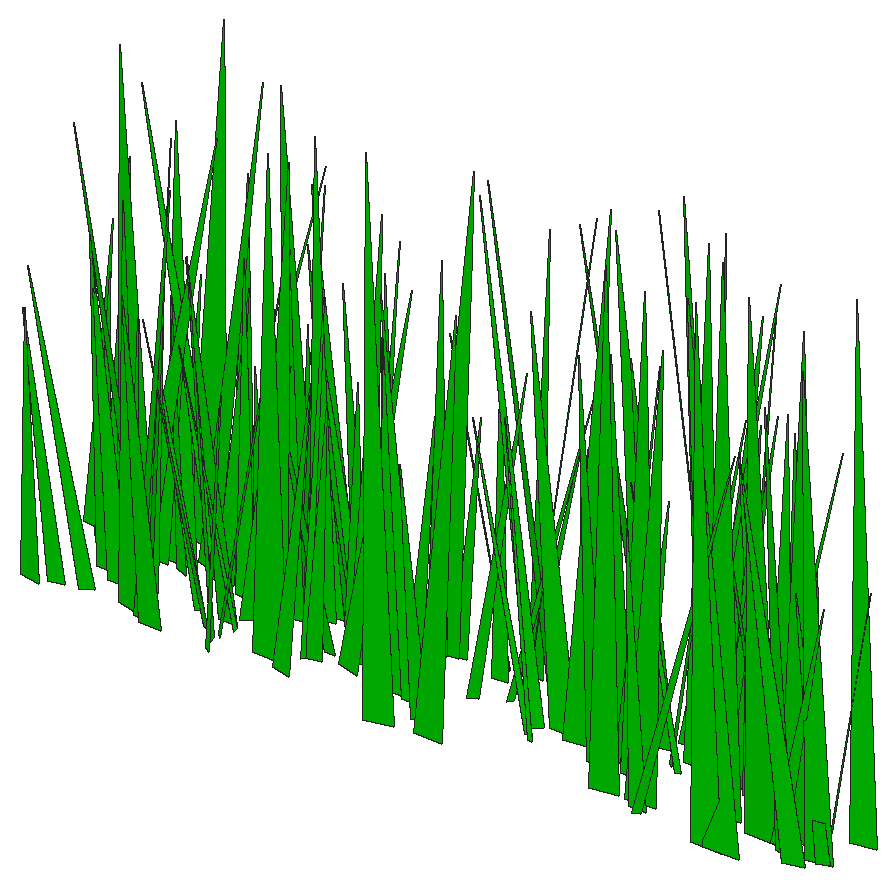
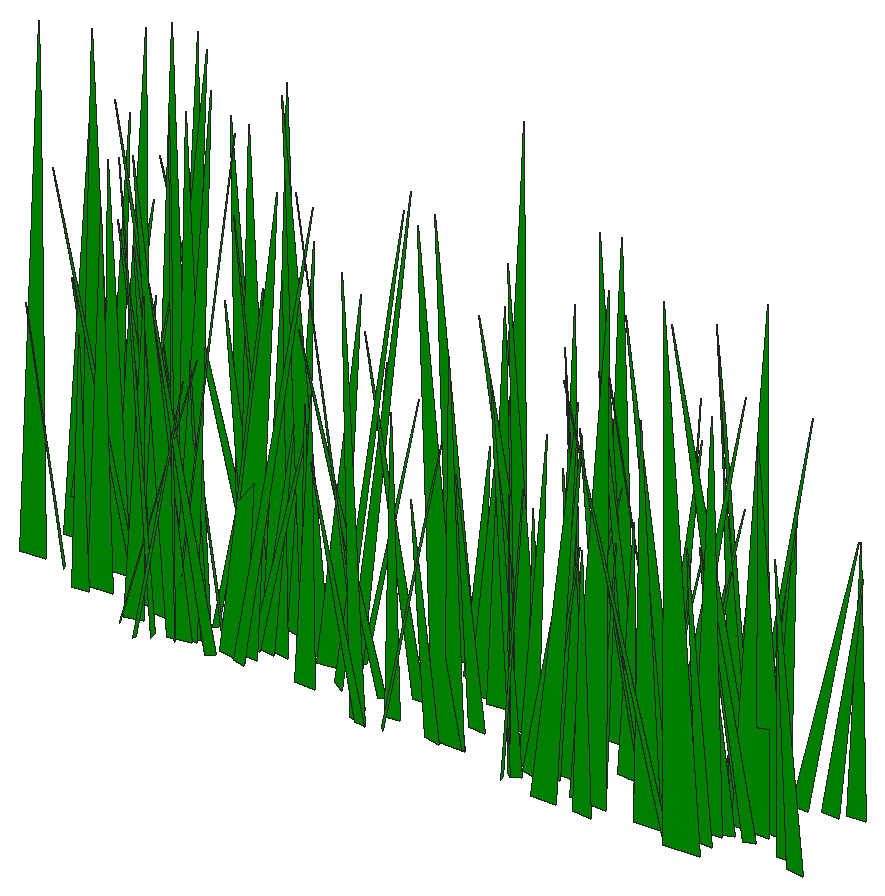
# SketchUp Ruby script. Lengths in inches.
U = 1.inch
M = Sketchup.active_model
def pt(a) = Geom::Point3d.new(a.map { |v| v * U })
def face(e, loops, mat)
  f = e.add_face(loops[0].map { |a| pt(a) })
  loops[1..].each { |l| e.add_face(l.map { |a| pt(a) }).erase! }
  f.material = f.back_material = mat if mat
  f
end
# faces: each face lists its corners as indices into pts; further lists are holes
def faces(e, pts, list, mat = nil) = list.each { |f| face(e, (f[0].is_a?(Array) ? f : [f]).map { |l| l.map { |i| pts[i] } }, mat) }
# xy, xz, yz: faces in a plane at the given z, y or x. An outline is a flat list of corners, or four numbers for a rectangle; further outlines are holes
def ring(l) = l.size == 4 ? [[l[0], l[1]], [l[2], l[1]], [l[2], l[3]], [l[0], l[3]]] : l.each_slice(2).to_a
def flat(e, list, mat, &to3) = list.each { |f| face(e, (f[0].is_a?(Array) ? f : [f]).map { |l| ring(l).map { |u, v| to3.(u, v) } }, mat) }
def xy(e, z, list, mat = nil) = flat(e, list, mat) { |x, y| [x, y, z] }
def xz(e, y, list, mat = nil) = flat(e, list, mat) { |x, z| [x, y, z] }
def yz(e, x, list, mat = nil) = flat(e, list, mat) { |y, z| [x, y, z] }
def lines(e, pts, list) = list.each { |a, b| e.add_line(pt(pts[a]), pt(pts[b])) }
# prism: a flat outline (further loops are holes) pulled along v
def prism(e, loops, v, mat = nil)
  f = face(e, loops, mat); d = Geom::Vector3d.new(v.map { |x| x * U })
  f.pushpull(f.normal.samedirection?(d) ? d.length : -d.length)
end
def box(e, o, s, mat = nil) = prism(e, [[o, [o[0] + s[0], o[1], o[2]], [o[0] + s[0], o[1] + s[1], o[2]], [o[0], o[1] + s[1], o[2]]]], [0, 0, s[2]], mat)
def at(x, y, z, deg = 0) = Geom::Transformation.translation(pt([x, y, z])) * Geom::Transformation.rotation(ORIGIN, Z_AXIS, deg.degrees)
def axes(o, x, y, z) = Geom::Transformation.new([*x, 0, *y, 0, *z, 0, *pt(o).to_a, 1])
def part(name) = M.definitions.add(name)
# library, detail: a bought-in or finely detailed component or shape, given as its bounding box
def library(name, o, s) = part(name).tap { |d| box(d.entities, o, s) }
def detail(e, o, s) = box(e.add_group.entities, o, s)
def put(e, d, t, mat = nil) = e.add_instance(d, t).tap { |i| i.material = mat if mat }
def group(e, t, mat = nil) = e.add_group.tap { |g| g.transformation = t; g.material = mat if mat }.entities
root = M.entities
M.materials.add("[Color G06]").color = [0, 204, 0]
c1 = part("fur_instance\#9")
p = [[0.8125,0,1.79],[0.67,-0.02,1.48],[0,-0.11,0],[0,0.11,0]]
faces(c1.entities,p,[[0,1,2,3]])
put(root,c1,axes([38.34,19.75,4.28],[1.95891,0.37402,1.38836],[2.78999,-0.28268,-0.04491],[-0.52265,-0.10717,4.96385]),"[Color G06]")
put(root,c1,axes([39.64,16.51,4.28],[-1.52361,0.36345,0.25373],[2.61074,0.21109,0.28432],[-0.07898,-0.03381,4.50325]),"[Color G06]")
put(root,c1,axes([38.93,16.22,4.28],[-0.56952,-0.43127,0.57193],[-3.10418,0.0833,0.3105],[0.27498,0.04708,4.6898]),"[Color G06]")
put(root,c1,axes([39.06,19.33,4.28],[-1.42932,0.30898,1.98096],[2.45507,0.22805,-0.12937],[0.7995,-0.14791,3.93877]),"[Color G06]")
put(root,c1,axes([40.55,16.76,4.28],[-2.69983,0.31266,0.21513],[2.24631,0.37498,0.36685],[-0.04649,-0.03915,5.23232]),"[Color G06]")
put(root,c1,axes([40.3,17.99,4.28],[-0.87197,-0.47369,1.57293],[-3.55457,0.12071,-0.2257],[0.10871,0.14748,5.2367]),"[Color G06]")
put(root,c1,axes([41.4,18.25,4.28],[-4.45741,-0.26061,1.16632],[-1.91035,0.62838,-0.17915],[0.6725,0.05768,7.22157]),"[Color G06]")
put(root,c1,axes([40.25,18.43,4.28],[-0.09806,0.66045,0.30571],[4.73938,0.01433,-0.16071],[0.11184,-0.0282,7.07841]),"[Color G06]")
put(root,c1,axes([41.07,17.56,4.28],[-1.7482,0.4674,0.05007],[3.35158,0.24382,-0.06691],[0.05519,-0.00125,5.64965]),"[Color G06]")
put(root,c1,axes([40.81,18.68,4.28],[-0.49228,-0.857,0.59789],[-6.15712,0.06978,0.16632],[0.1431,0.05435,9.21324]),"[Color G06]")
put(root,c1,axes([40.43,19.22,4.28],[2.5384,-0.26237,0.54487],[-1.90667,-0.35426,0.24589],[-0.19387,0.04878,4.71595]),"[Color G06]")
put(root,c1,axes([41.23,18.02,4.28],[-1.85599,-0.24708,1.92715],[-1.99358,0.28821,-0.04391],[0.90989,0.12747,3.83481]),"[Color G06]")
put(root,c1,axes([41.75,19.51,4.28],[-1.24285,0.66776,0.86536],[4.81651,0.17632,-0.1775],[0.26115,-0.07394,7.39206]),"[Color G06]")
put(root,c1,axes([43.23,19.48,4.28],[-4.84602,0.32177,0.63164],[2.29807,0.67832,-0.31162],[0.4712,0.00101,8.01585]),"[Color G06]")
put(root,c1,axes([41.18,19.29,4.28],[-1.69214,0.27015,2.63551],[2.24982,0.29982,-0.30376],[1.342,-0.16201,3.83239]),"[Color G06]")
put(root,c1,axes([41.35,20.09,4.28],[2.34675,-0.3019,0.9507],[-2.16892,-0.33709,-0.33754],[-0.62251,0.03639,4.76001]),"[Color G06]")
put(root,c1,axes([42.01,19.19,4.28],[2.26278,0.18183,2.32042],[1.64416,-0.3544,-0.39131],[-1.18635,-0.14435,3.88355]),"[Color G06]")
put(root,c1,axes([42.12,16.68,4.28],[-2.70949,-0.45059,2.28251],[-3.37619,0.41036,0.35371],[1.17259,0.14038,6.2926]),"[Color G06]")
put(root,c1,axes([41.65,20.79,4.28],[1.33113,-0.81223,1.77595],[-5.94381,-0.18473,0.24621],[-0.10089,0.16669,8.92648]),"[Color G06]")
put(root,c1,axes([41.84,17.84,4.28],[1.19606,-0.45598,1.69007],[-3.45629,-0.16512,0.34634],[-0.15877,0.15943,5.19228]),"[Color G06]")
put(root,c1,axes([41.1,18.37,4.28],[4.40341,-0.43608,0.87741],[-3.16509,-0.61465,0.38893],[-0.32652,0.07711,8.06267]),"[Color G06]")
put(root,c1,axes([42.35,17.3,4.28],[4.85019,0.01314,2.67787],[0.02729,-0.72059,0.29568],[-1.79399,0.02456,7.2443]),"[Color G06]")
put(root,c1,axes([43.24,16.22,4.28],[-0.87022,-0.51976,0.36112],[-3.73513,0.12102,-0.09555],[-0.00745,0.03484,5.71976]),"[Color G06]")
put(root,c1,axes([43.75,17.81,4.28],[-2.45306,0.15496,0.50085],[1.13781,0.34263,0.27026],[0.22937,-0.04239,4.01585]),"[Color G06]")
put(root,c1,axes([42.64,16.42,4.28],[4.36002,0.21291,2.09252],[1.54919,-0.63713,0.23681],[-1.37534,-0.0427,6.90034]),"[Color G06]")
put(root,c1,axes([42.4375,19.85,4.28],[4.31135,0.4729,1.86217],[3.49232,-0.61479,-0.12612],[-0.92568,-0.11689,8.19722]),"[Color G06]")
put(root,c1,axes([44.54,17.125,4.28],[-3.14894,-0.1574,0.31267],[-1.12711,0.44007,0.09201],[0.21771,0.00174,4.99869]),"[Color G06]")
put(root,c1,axes([43.3,20.26,4.28],[0.08313,-0.59845,1.88169],[-4.46944,-0.00464,0.2715],[0.16492,0.17588,6.40959]),"[Color G06]")
put(root,c1,axes([43.33,19.48,4.28],[2.06213,-0.38234,0.88474],[-2.78108,-0.29203,-0.01799],[-0.36558,0.06495,5.12747]),"[Color G06]")
put(root,c1,axes([44.82,17.76,4.28],[-2.41213,-0.42614,1.13599],[-3.13112,0.33879,-0.25159],[0.33585,0.09794,5.8133]),"[Color G06]")
put(root,c1,axes([42.34,20.6,4.28],[4.82023,0.21456,0.31853],[1.54643,-0.67197,-0.27848],[-0.14619,-0.0338,7.55719]),"[Color G06]")
put(root,c1,axes([45.26,17.54,4.28],[-3.04685,0.01316,0.40509],[0.10791,0.42598,0.22314],[0.26595,-0.02206,4.55045]),"[Color G06]")
put(root,c1,axes([44.35,19.14,4.28],[-2.12981,0.39609,1.63645],[2.9171,0.31882,-0.3842],[0.87036,-0.09933,5.29217]),"[Color G06]")
put(root,c1,axes([45.09,16.72,4.28],[-3.91462,-0.00975,1.92647],[-0.00389,0.57403,0.31609],[1.29087,-0.02784,5.84307]),"[Color G06]")
put(root,c1,axes([45.24,19.9,4.28],[2.08173,0.19623,2.18823],[1.64305,-0.33458,-0.04489],[-1.19342,-0.11835,3.7552]),"[Color G06]")
put(root,c1,axes([45.15,20.93,4.28],[0.83363,-0.3955,0.68011],[-2.85909,-0.12063,-0.23026],[-0.2777,0.05467,4.41231]),"[Color G06]")
put(root,c1,axes([44.49,18.98,4.28],[2.85829,-0.00608,0.616],[-0.06124,-0.40231,0.17877],[-0.4099,0.01773,4.26868]),"[Color G06]")
put(root,c1,axes([45.42,20.3,4.28],[-0.5313,-0.84193,0.42446],[-6.04346,0.07468,0.1193],[0.1045,0.03847,9.05785]),"[Color G06]")
put(root,c1,axes([45.5,18.45,4.28],[0.37967,-0.40285,0.55943],[-2.90539,-0.0562,-0.24423],[-0.21205,0.04868,4.34805]),"[Color G06]")
put(root,c1,axes([45.36,16.16,4.28],[2.57846,0.10869,1.42387],[0.84403,-0.38058,-0.07686],[-0.89599,-0.04572,4.0252]),"[Color G06]")
put(root,c1,axes([45.19,18.2,4.28],[3.78591,-0.29659,1.20831],[-2.13398,-0.53876,-0.25613],[-0.78968,0.03398,6.48508]),"[Color G06]")
put(root,c1,axes([46.53,20.9375,4.28],[-1.84614,-0.60322,0.67971],[-4.33773,0.26043,0.23321],[0.32259,0.04972,7.02562]),"[Color G06]")
put(root,c1,axes([46.15,19.06,4.28],[2.0082,-0.40327,2.09576],[-3.06438,-0.30977,-0.28826],[-0.96913,0.14386,5.25422]),"[Color G06]")
put(root,c1,axes([45.09,17.04,4.28],[4.17661,0.07004,1.01495],[0.54368,-0.58853,-0.33206],[-0.64642,-0.04245,6.27845]),"[Color G06]")
put(root,c1,axes([46,19.53,4.28],[4.40701,0.14624,2.338],[1.14607,-0.64873,-0.16432],[-1.49445,-0.06626,6.76853]),"[Color G06]")
put(root,c1,axes([47.08,19.82,4.28],[-3.36827,0.26388,1.57482],[1.96425,0.48662,0.01755],[0.91268,-0.07345,5.77418]),"[Color G06]")
put(root,c1,axes([47.24,20.13,4.28],[-2.53432,-0.16838,0.68261],[-1.2217,0.35815,0.01676],[0.4172,0.02596,4.19565]),"[Color G06]")
put(root,c1,axes([46.82,19.5,4.28],[-3.01113,0.51935,3.32616],[4.15815,0.45328,0.27819],[1.23852,-0.25914,7.15268]),"[Color G06]")
put(root,c1,axes([47.8,20.01,4.28],[-2.41641,0.27132,0.71727],[1.99222,0.33658,0.36666],[0.21694,-0.0688,4.62221]),"[Color G06]")
put(root,c1,axes([47.0625,16.85,4.28],[-0.54366,-0.72478,2.86792],[-5.53489,0.08313,0.06971],[0.24903,0.2654,7.81024]),"[Color G06]")
put(root,c1,axes([48.19,18.14,4.28],[-2.71049,-0.26301,0.25504],[-1.89354,0.3771,-0.27789],[0.0335,0.03488,4.92749]),"[Color G06]")
put(root,c1,axes([46.99,17.0625,4.28],[2.85977,-0.6436,2.13179],[-4.75343,-0.4161,-0.18703],[-0.86105,0.15953,8.11275]),"[Color G06]")
put(root,c1,axes([48.05,19.76,4.28],[-2.05197,-0.41979,1.55318],[-3.12717,0.29822,0.03058],[0.60289,0.11807,5.44502]),"[Color G06]")
put(root,c1,axes([48.26,20.68,4.28],[-3.17128,0.00424,1.49021],[-0.00014,0.46337,-0.15194],[0.99755,0.01353,4.7375]),"[Color G06]")
put(root,c1,axes([47.875,19.63,4.28],[0.1676,-0.41515,0.29631],[-2.98164,-0.02225,0.18557],[0.1131,0.02855,4.45281]),"[Color G06]")
put(root,c1,axes([47.77,17.54,4.28],[3.75891,-0.13891,1.86612],[-0.96117,-0.55228,-0.39788],[-1.27573,0.00681,5.79826]),"[Color G06]")
put(root,c1,axes([48.24,20.39,4.28],[2.77009,0.09919,1.88209],[0.67892,-0.42419,0.33611],[-1.27705,-0.01035,4.26119]),"[Color G06]")
put(root,c1,axes([47.76,16.47,4.28],[1.81356,0.35978,1.22968],[2.6936,-0.2539,-0.34031],[-0.27939,-0.11249,4.70109]),"[Color G06]")
put(root,c1,axes([48.04,17.58,4.28],[1.67917,-0.34109,0.71224],[-2.4594,-0.23975,-0.23761],[-0.40207,0.042,4.42797]),"[Color G06]")
put(root,c1,axes([47.98,20.375,4.28],[3.90037,-0.18362,1.91403],[-1.36867,-0.57006,-0.05224],[-1.22503,0.05228,6.1524]),"[Color G06]")
put(root,c1,axes([49.23,18.22,4.28],[3.23938,-0.54112,1.72848],[-3.94216,-0.46863,-0.34999],[-0.92476,0.1022,7.54678]),"[Color G06]")
put(root,c1,axes([49.14,17.75,4.28],[3.1422,0.45614,0.89658],[3.31747,-0.43799,-0.37279],[-0.2335,-0.08454,6.76886]),"[Color G06]")
put(root,c1,axes([50.48,20.07,4.28],[2.36878,0.44894,2.41421],[3.46328,-0.35796,0.05622],[-0.98993,-0.17807,5.97357]),"[Color G06]")
put(root,c1,axes([50.86,17.49,4.28],[-1.68936,0.56568,1.84491],[4.19903,0.24897,-0.18054],[0.59021,-0.15212,6.56521]),"[Color G06]")
put(root,c1,axes([50.55,18.94,4.28],[0.93922,0.38239,0.57742],[2.76785,-0.13145,-0.05698],[-0.08879,-0.0527,4.33176]),"[Color G06]")
put(root,c1,axes([51.71,17.39,4.28],[-3.31939,0.38103,1.36712],[2.76636,0.47585,-0.23179],[0.80653,-0.06394,6.42159]),"[Color G06]")
put(root,c1,axes([50.63,20.13,4.28],[2.7096,-0.71167,0.94544],[-5.12792,-0.38143,-0.15431],[-0.38833,0.07111,8.63464]),"[Color G06]")
put(root,c1,axes([51.17,20.22,4.28],[1.29623,0.3553,0.21932],[2.53743,-0.18188,0.34812],[-0.27419,-0.00343,4.2584]),"[Color G06]")
put(root,c1,axes([51.73,15.89,4.28],[3.62593,-0.59838,3.94841],[-4.67185,-0.56928,-0.32728],[-1.88863,0.25939,8.39003]),"[Color G06]")
put(root,c1,axes([52.71,20.56,4.28],[-3.54835,-0.06477,0.63017],[-0.47873,0.49784,-0.14355],[0.40537,0.021,5.34659]),"[Color G06]")
put(root,c1,axes([52.51,16.75,4.28],[-1.07609,0.33652,1.06807],[2.51593,0.14676,0.35037],[0.06809,-0.10445,3.93356]),"[Color G06]")
put(root,c1,axes([52.85,19.94,4.28],[-2.33183,0.29174,1.99998],[2.24657,0.3569,-0.12964],[1.05863,-0.11478,4.68043]),"[Color G06]")
put(root,c1,axes([53.52,20.69,4.28],[3.72225,0.39183,2.51322],[2.94513,-0.55577,0.21033],[-1.43161,-0.12456,6.96718]),"[Color G06]")
put(root,c1,axes([53.35,16.09,4.28],[2.26934,-0.57922,1.76717],[-4.30205,-0.31953,0.30928],[-0.37917,0.15881,7.06737]),"[Color G06]")
put(root,c1,axes([52.91,18.66,4.28],[3.64207,-0.22641,0.71099],[-1.61793,-0.51212,-0.22113],[-0.49487,0.00801,5.95567]),"[Color G06]")
put(root,c1,axes([55.22,19.43,4.28],[-5.28888,-0.23345,1.83293],[-1.76747,0.75207,-0.3885],[1.08759,0.08694,8.28207]),"[Color G06]")
put(root,c1,axes([53.41,20.73,4.28],[2.3865,0.22497,0.35028],[1.62232,-0.33344,-0.08883],[-0.16073,-0.02519,4.30444]),"[Color G06]")
put(root,c1,axes([55.36,18.46,4.28],[-5.30138,0.20809,2.05154],[1.58672,0.75936,0.31097],[1.26226,-0.08061,8.22533]),"[Color G06]")
put(root,c1,axes([55.43,18,4.28],[-3.30676,0.10063,0.45842],[0.70713,0.46281,-0.27701],[0.3389,0.01625,5.05093]),"[Color G06]")
put(root,c1,axes([53.75,20.1,4.28],[5.47348,0.04989,1.65244],[0.40944,-0.77755,-0.33253],[-1.08756,-0.04163,8.19124]),"[Color G06]")
put(root,c1,axes([55.68,17.76,4.28],[-3.29571,0.05434,1.42652],[0.35496,0.47836,-0.26149],[0.96792,0.0096,4.9531]),"[Color G06]")
put(root,c1,axes([56.14,18.67,4.28],[-2.42821,0.56729,0.22367],[4.06304,0.33923,-0.308],[0.25368,-0.00317,7.07424]),"[Color G06]")
put(root,c1,axes([53.83,19.19,4.28],[3.96685,-0.11465,0.04786],[-0.82045,-0.55281,-0.22952],[-0.0625,-0.02006,6.05041]),"[Color G06]")
put(root,c1,axes([55.99,19.99,4.28],[0.03715,-0.42086,1.73979],[-3.23273,-0.01062,-0.14104],[-0.11545,0.16206,4.50888]),"[Color G06]")
put(root,c1,axes([56.34,19.51,4.28],[2.24372,-0.21543,1.90281],[-1.72909,-0.34294,0.09408],[-1.00893,0.10864,4.07037]),"[Color G06]")
put(root,c1,axes([58.27,20.12,4.28],[-4.99035,-0.30863,1.31117],[-2.22823,0.70553,0.13389],[0.83863,0.03802,8.158]),"[Color G06]")
put(root,c1,axes([58.34,19.29,4.28],[-2.93667,0.14549,0.19818],[1.04069,0.4099,-0.12185],[0.15222,0.00453,4.65627]),"[Color G06]")
put(root,c1,axes([56.82,18.45,4.28],[4.36748,-0.54329,2.55111],[-4.07093,-0.63278,0.08759],[-1.23306,0.16479,8.74686]),"[Color G06]")
put(root,c1,axes([58.03,19.16,4.28],[1.21212,-0.26043,2.36367],[-2.17463,-0.2275,-0.38846],[-1.12252,0.15952,3.30487]),"[Color G06]")
put(root,c1,axes([57.85,19.02,4.28],[0.06914,0.5858,1.40469],[4.29518,-0.01815,0.39715],[-0.2877,-0.13015,6.2669]),"[Color G06]")
put(root,c1,axes([58.01,17.83,4.28],[2.48356,0.41672,3.20383],[3.37809,-0.40108,0.14345],[-1.454,-0.22005,5.80566]),"[Color G06]")
put(root,c1,axes([58.59,19.6875,4.28],[-2.14968,0.72718,0.90283],[5.24956,0.29826,0.3239],[0.02855,-0.0894,8.42388]),"[Color G06]")
put(root,c1,axes([58.63,19.98,4.28],[-0.89372,-0.57813,1.04233],[-4.20343,0.121,-0.34098],[-0.07927,0.10172,6.32956]),"[Color G06]")
put(root,c1,axes([58.36,18.32,4.28],[4.41497,-0.04117,1.7638],[-0.35482,-0.63614,0.27826],[-1.16361,0.03778,6.60738]),"[Color G06]")
put(root,c1,axes([60.08,18.9,4.28],[-3.00719,0.09361,0.57247],[0.66842,0.42272,-0.09714],[0.38802,-0.00272,4.60407]),"[Color G06]")
put(root,c1,axes([59.13,16.76,4.28],[3.26089,-0.60286,3.16183],[-4.60746,-0.49404,-0.20654],[-1.39196,0.22298,8.09074]),"[Color G06]")
put(root,c1,axes([60.6875,20.08,4.28],[-5.707,-0.12377,2.04048],[-0.86422,0.81827,0.30223],[1.38014,0.00061,8.62678]),"[Color G06]")
put(root,c1,axes([59.41,17.92,4.28],[1.07811,-0.71862,2.28956],[-5.37098,-0.15365,0.10955],[-0.23894,0.21125,7.86815]),"[Color G06]")
put(root,c1,axes([59.76,19.82,4.28],[2.55014,0.21465,1.36185],[1.54524,-0.37581,0.34117],[-0.90116,-0.03697,4.43882]),"[Color G06]")
put(root,c1,axes([60.39,19.97,4.28],[-3.87564,-0.63196,2.57575],[-4.66397,0.57,0.38961],[1.32524,0.15787,8.90387]),"[Color G06]")
put(root,c1,axes([60.48,16.58,4.28],[-1.48452,0.36588,0.87499],[2.66191,0.21309,-0.14782],[0.37583,-0.0641,4.50318]),"[Color G06]")
put(root,c1,axes([59.65,19.13,4.28],[2.74816,0.08677,0.81298],[0.64622,-0.38978,-0.1007],[-0.51522,-0.02608,4.21009]),"[Color G06]")
put(root,c1,axes([59.21,20.27,4.28],[3.70981,-0.19303,0.82148],[-1.42697,-0.51958,0.36986],[-0.42661,0.05938,5.90642]),"[Color G06]")
put(root,c1,axes([59.97,17.2,4.28],[0.9415,0.45471,0.76817],[3.29907,-0.127,-0.39638],[0.11557,-0.07902,5.05713]),"[Color G06]")
put(root,c1,axes([60.47,19.47,4.28],[-1.06529,0.74614,2.88125],[5.65898,0.16639,-0.27617],[0.56841,-0.25816,8.14939]),"[Color G06]")
put(root,c1,axes([61.52,20.82,4.28],[-3.14178,0.03636,0.66378],[0.26774,0.44236,0.0475],[0.43993,-0.00958,4.71152]),"[Color G06]")
put(root,c1,axes([60.61,20.15,4.28],[5.23515,0.13378,3.43173],[0.94369,-0.79683,0.35257],[-2.30261,-0.02242,7.94679]),"[Color G06]")
put(root,c1,axes([60.35,16.875,4.28],[2.325,-0.66303,1.19662],[-4.8019,-0.32961,-0.13922],[-0.43629,0.09451,7.90917]),"[Color G06]")
put(root,c1,axes([62.39,20.38,4.28],[-3.49734,-0.0514,0.06164],[-0.36761,0.48761,0.1207],[0.04947,-0.0106,5.25459]),"[Color G06]")
put(root,c1,axes([60.43,20.125,4.28],[3.7071,-0.50172,1.50865],[-3.68359,-0.52399,0.2003],[-0.629,0.11167,7.71845]),"[Color G06]")
put(root,c1,axes([59.9375,19.76,4.28],[5.72609,-0.12126,1.19157],[-0.87076,-0.80612,-0.07658],[-0.79596,0.00956,8.65584]),"[Color G06]")
put(root,c1,axes([61.1875,20.4,4.28],[4.95721,0.01524,2.34929],[0.06326,-0.72493,0.24191],[-1.5744,0.01884,7.40676]),"[Color G06]")
put(root,c1,axes([62.21,19.99,4.28],[-1.99807,0.42351,1.29378],[3.09878,0.29047,-0.23269],[0.60904,-0.08849,5.42842]),"[Color G06]")
put(root,c1,axes([62.48,19.6,4.28],[2.89938,-0.15269,2.78344],[-1.26325,-0.47242,-0.03779],[-1.75261,0.0879,4.63193]),"[Color G06]")
put(root,c1,axes([61.65,19.375,4.28],[2.18555,0.46163,1.44747],[3.41507,-0.31205,-0.08586],[-0.48418,-0.11724,5.92812]),"[Color G06]")
put(root,c1,axes([61.55,17.91,4.28],[2.77347,-0.066,0.7418],[-0.46431,-0.39289,-0.13765],[-0.50473,-0.00122,4.20282]),"[Color G06]")
put(root,c1,axes([61.35,19.26,4.28],[3.52837,0.33857,1.15226],[2.49172,-0.49689,-0.27153],[-0.5299,-0.08209,6.39556]),"[Color G06]")
put(root,c1,axes([60.6,16.4,4.28],[4.63166,-0.13552,0.15531],[-0.97344,-0.64591,0.09935],[-0.08804,0.01205,7.07241]),"[Color G06]")
put(root,c1,axes([62.68,19.11,4.28],[-0.08661,0.5307,1.07228],[3.86965,0.00783,0.25312],[-0.15599,-0.10047,5.68383]),"[Color G06]")
put(root,c1,axes([62.61,17.7,4.28],[1.78674,-0.80102,2.43936],[-5.93423,-0.26474,-0.2771],[-0.66796,0.20926,8.98679]),"[Color G06]")
put(root,c1,axes([63.89,16.08,4.28],[-2.46961,0.78876,0.65914],[5.66987,0.34554,-0.04692],[0.20531,-0.0546,9.22444]),"[Color G06]")
put(root,c1,axes([63.36,16.06,4.28],[-3.67266,0.5956,2.73508],[4.43381,0.54651,-0.37214],[1.39047,-0.1695,8.41082]),"[Color G06]")
put(root,c1,axes([64.14,18.02,4.28],[-3.03557,-0.16762,0.86775],[-1.25089,0.4274,-0.29038],[0.46621,0.05534,4.871]),"[Color G06]")
put(root,c1,axes([64.01,19.26,4.28],[-0.83786,-0.56445,1.54734],[-4.15202,0.12891,0.38004],[0.46615,0.13369,6.16628]),"[Color G06]")
put(root,c1,axes([64.31,17.42,4.28],[-1.18744,-0.77868,2.64049],[-5.84629,0.17274,-0.02088],[0.35317,0.2414,8.53248]),"[Color G06]")
put(root,c1,axes([64.24,18.21,4.28],[-1.13217,0.56172,2.7087],[4.36265,0.18306,-0.2878],[0.69188,-0.23512,6.24717]),"[Color G06]")
put(root,c1,axes([64.45,19.62,4.28],[-0.11019,-0.40357,0.4556],[-2.90404,0.01799,0.2617],[0.18751,0.04147,4.32062]),"[Color G06]")
put(root,c1,axes([63.31,18.5,4.28],[4.52507,-0.06039,0.59629],[-0.45711,-0.63205,0.39482],[-0.37122,0.0421,6.78247]),"[Color G06]")
put(root,c1,axes([65.89,16.8125,4.28],[-2.61979,0.47663,0.40864],[3.42892,0.36419,0.30684],[0.00287,-0.04768,6.42908]),"[Color G06]")
put(root,c1,axes([65.34,17.09,4.28],[-3.5003,-0.4256,2.26949],[-3.16136,0.51881,0.28506],[1.27542,0.11795,6.93502]),"[Color G06]")
put(root,c1,axes([65.16,17.9,4.28],[0.79301,-0.8244,1.11673],[-5.95903,-0.10982,0.13936],[-0.00618,0.105,8.91397]),"[Color G06]")
put(root,c1,axes([64.875,17.42,4.28],[2.20011,-0.2978,0.15316],[-2.13808,-0.3064,0.16744],[0.00459,0.02116,4.57954]),"[Color G06]")
put(root,c1,axes([66.54,17.34,4.28],[-1.88008,0.2964,0.92394],[2.19802,0.26337,0.28487],[0.26253,-0.08245,4.23163]),"[Color G06]")
put(root,c1,axes([66.39,17.35,4.28],[2.97887,-0.51103,3.64644],[-4.06906,-0.47642,-0.24468],[-1.68097,0.24764,7.05419]),"[Color G06]")
put(root,c1,axes([65.61,18.89,4.28],[2.82495,0.03024,0.76738],[0.18306,-0.3997,0.30404],[-0.52644,0.02328,4.22359]),"[Color G06]")
put(root,c1,axes([66.75,18.89,4.28],[-4.25662,0.47758,3.56763],[3.7623,0.64487,0.11041],[1.80909,-0.2174,8.16468]),"[Color G06]")
